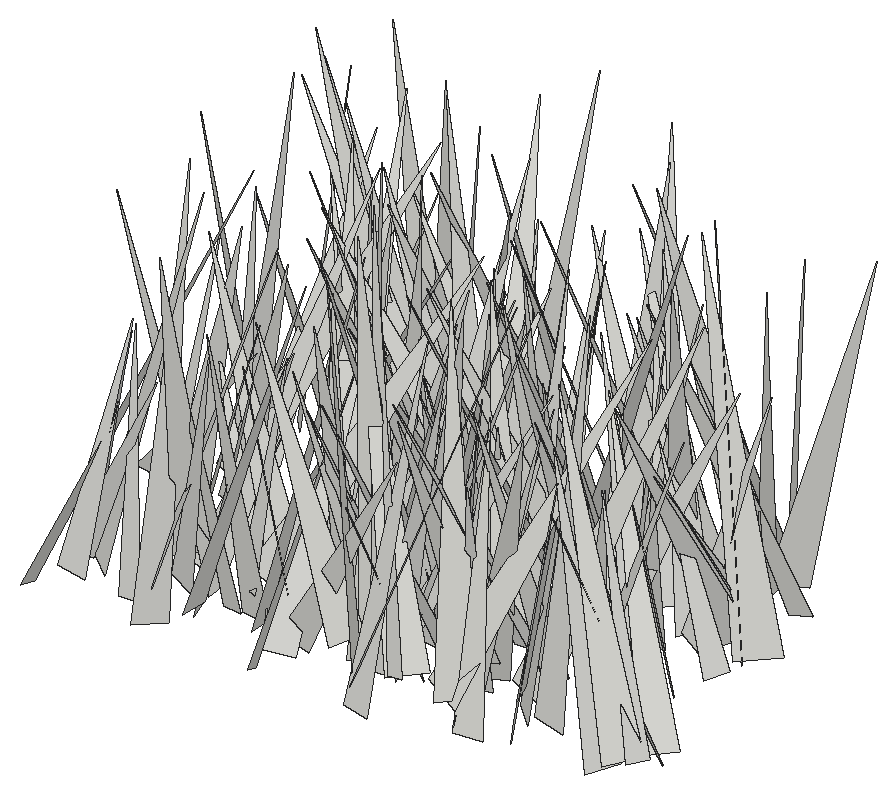
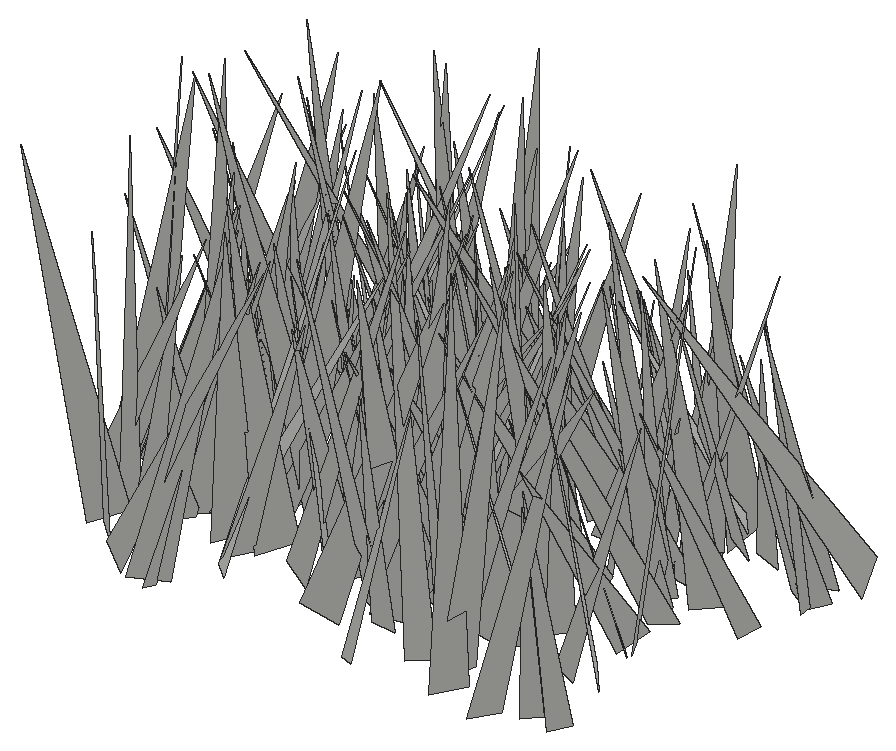
# SketchUp Ruby script. Lengths in inches.
U = 1.inch
M = Sketchup.active_model
def pt(a) = Geom::Point3d.new(a.map { |v| v * U })
def face(e, loops, mat)
  f = e.add_face(loops[0].map { |a| pt(a) })
  loops[1..].each { |l| e.add_face(l.map { |a| pt(a) }).erase! }
  f.material = f.back_material = mat if mat
  f
end
# faces: each face lists its corners as indices into pts; further lists are holes
def faces(e, pts, list, mat = nil) = list.each { |f| face(e, (f[0].is_a?(Array) ? f : [f]).map { |l| l.map { |i| pts[i] } }, mat) }
# xy, xz, yz: faces in a plane at the given z, y or x. An outline is a flat list of corners, or four numbers for a rectangle; further outlines are holes
def ring(l) = l.size == 4 ? [[l[0], l[1]], [l[2], l[1]], [l[2], l[3]], [l[0], l[3]]] : l.each_slice(2).to_a
def flat(e, list, mat, &to3) = list.each { |f| face(e, (f[0].is_a?(Array) ? f : [f]).map { |l| ring(l).map { |u, v| to3.(u, v) } }, mat) }
def xy(e, z, list, mat = nil) = flat(e, list, mat) { |x, y| [x, y, z] }
def xz(e, y, list, mat = nil) = flat(e, list, mat) { |x, z| [x, y, z] }
def yz(e, x, list, mat = nil) = flat(e, list, mat) { |y, z| [x, y, z] }
def lines(e, pts, list) = list.each { |a, b| e.add_line(pt(pts[a]), pt(pts[b])) }
# prism: a flat outline (further loops are holes) pulled along v
def prism(e, loops, v, mat = nil)
  f = face(e, loops, mat); d = Geom::Vector3d.new(v.map { |x| x * U })
  f.pushpull(f.normal.samedirection?(d) ? d.length : -d.length)
end
def box(e, o, s, mat = nil) = prism(e, [[o, [o[0] + s[0], o[1], o[2]], [o[0] + s[0], o[1] + s[1], o[2]], [o[0], o[1] + s[1], o[2]]]], [0, 0, s[2]], mat)
def at(x, y, z, deg = 0) = Geom::Transformation.translation(pt([x, y, z])) * Geom::Transformation.rotation(ORIGIN, Z_AXIS, deg.degrees)
def axes(o, x, y, z) = Geom::Transformation.new([*x, 0, *y, 0, *z, 0, *pt(o).to_a, 1])
def part(name) = M.definitions.add(name)
# library, detail: a bought-in or finely detailed component or shape, given as its bounding box
def library(name, o, s) = part(name).tap { |d| box(d.entities, o, s) }
def detail(e, o, s) = box(e.add_group.entities, o, s)
def put(e, d, t, mat = nil) = e.add_instance(d, t).tap { |i| i.material = mat if mat }
def group(e, t, mat = nil) = e.add_group.tap { |g| g.transformation = t; g.material = mat if mat }.entities
root = M.entities
c1 = part("fur_instance\#9")
p = [[0.8125,0,1.79],[0.67,-0.02,1.48],[0,-0.11,0],[0,0.11,0]]
faces(c1.entities,p,[[0,1,2,3]])
put(root,c1,axes([118.43,200.45,-27.1],[6.55283,1.12937,1.12544],[0.97488,-6.60494,0.95181],[-1.26162,0.76214,6.58096]))
put(root,c1,axes([128.43,203.72,-27.1],[1.50349,-5.86365,0.5049],[-5.82358,-1.55753,-0.74685],[-0.85041,0.2992,6.00709]))
put(root,c1,axes([121.35,202.26,-28.22],[2.07826,-5.21506,0.82935],[-4.82149,-1.51054,2.58366],[2.15357,1.65083,4.98405]))
put(root,c1,axes([123.91,201.99,-27.1],[-5.32926,2.77314,1.19327],[2.9808,5.21718,1.1879],[0.47858,-1.6143,5.88899]))
put(root,c1,axes([126.07,203.33,-28.22],[-2.66612,-3.28273,0.28859],[-3.19335,2.6653,0.81637],[0.81369,-0.29607,4.14946]))
put(root,c1,axes([126.01,199.82,-28.22],[2.11808,6.39246,0.96016],[6.39192,-2.22182,0.69185],[-0.96378,-0.68681,6.6986]))
put(root,c1,axes([131.1,202.04,-28.22],[4.62058,2.87983,1.50344],[3.15499,-4.60106,-0.88304],[-0.77446,-1.56215,5.37246]))
put(root,c1,axes([136.55,201.3,-27.1],[-5.76808,3.66085,1.08427],[3.77252,5.76709,0.59739],[0.58783,-1.08949,6.80556]))
put(root,c1,axes([129.43,201.09,-27.1],[-5.69,4.35692,2.08043],[4.49689,5.95288,-0.16772],[1.75752,-1.1258,7.16454]))
put(root,c1,axes([119.28,202.8125,-28.22],[-0.73911,-5.79285,1.55471],[-5.99778,0.70592,-0.22109],[-0.03032,1.57006,5.83563]))
put(root,c1,axes([125.12,201.11,-28.22],[-6.49961,-2.89491,2.26898],[-3.37847,6.5202,-1.35892],[1.4542,2.20912,6.98418]))
put(root,c1,axes([115.99,203.56,-27.1],[4.78165,-4.93816,1.39024],[-4.88475,-4.96331,-0.82896],[-1.56762,0.40313,6.82367]))
put(root,c1,axes([112.33,201.38,-28.22],[0.08637,4.97569,1.67082],[5.15736,0.22998,-0.95146],[0.97504,-1.65717,4.88463]))
put(root,c1,axes([130.11,200.84,-28.22],[-0.17119,5.69768,1.30234],[5.83131,0.07859,0.42267],[-0.39436,-1.31119,5.68456]))
put(root,c1,axes([135.11,201.98,-28.22],[-5.24229,2.67543,1.59997],[2.88849,5.34612,0.52444],[1.17239,-1.20849,5.86212]))
put(root,c1,axes([125.73,200.1,-27.1],[6.75975,3.62956,0.52461],[3.54067,-6.74583,1.04905],[-0.95528,0.68056,7.60048]))
put(root,c1,axes([136.04,203.83,-28.22],[-3.22391,-4.50813,0.36238],[-4.51102,3.23719,0.13952],[0.32445,0.21334,5.54053]))
put(root,c1,axes([115.06,201.15,-28.22],[0.59003,4.76484,1.13067],[4.77949,-0.80843,0.91275],[-1.06703,-0.9864,4.71367]))
put(root,c1,axes([117.36,202.06,-28.22],[4.51759,1.55237,1.02195],[1.60919,-4.61101,-0.10928],[-0.92991,-0.4377,4.77562]))
put(root,c1,axes([115.81,203.07,-28.22],[-0.90647,-5.11686,1.80724],[-5.12934,1.40604,1.40817],[1.7715,1.45288,5.00209]))
put(root,c1,axes([111.72,202.58,-28.22],[2.80159,-3.67069,0.58517],[-3.61323,-2.51742,1.50747],[0.87232,1.36159,4.36468]))
put(root,c1,axes([129.96,205.05,-27.1],[-4.86076,-4.47494,0.06756],[-4.36579,4.76306,1.38194],[0.98465,-0.972,6.46083]))
put(root,c1,axes([127.02,201.38,-27.1],[-4.60264,5.20733,0.96805],[5.29634,4.53648,0.77902],[0.04773,-1.24166,6.90606]))
put(root,c1,axes([111.87,202.94,-28.22],[5.07227,1.20948,1.05659],[1.39553,-5.05165,-0.91676],[-0.7948,-1.15114,5.13326]))
put(root,c1,axes([128.25,203.69,-28.22],[1.54796,-4.76639,0.70367],[-4.81569,-1.50748,0.38266],[0.1508,0.78667,4.99682]))
put(root,c1,axes([118.28,202.76,-28.22],[-1.858,-4.3991,1.45242],[-4.62148,1.65138,-0.9103],[-0.32175,1.68364,4.68782]))
put(root,c1,axes([127.35,203.25,-27.1],[-2.08811,-4.65792,0.59921],[-4.45757,1.75934,-1.85749],[-1.47829,1.27435,4.7546]))
put(root,c1,axes([124.63,203.15,-27.1],[-4.81324,5.46383,3.73935],[6.29264,5.21276,0.48307],[2.05886,-3.15867,7.26549]))
put(root,c1,axes([121.36,199.98,-28.22],[4.83042,2.64277,1.00625],[2.0268,-4.62442,2.4159],[-1.97202,1.72053,4.9478]))
put(root,c1,axes([124.89,203.09,-28.22],[5.25974,-3.61511,1.15521],[-3.73911,-5.27428,0.51907],[-0.65007,1.0869,6.36116]))
put(root,c1,axes([126.47,200.94,-27.1],[1.43872,7.93621,2.15807],[7.82752,-1.99366,2.11323],[-2.52399,-1.65906,7.7838]))
put(root,c1,axes([136.99,201.56,-27.1],[-4.67353,1.04438,0.03845],[1.02272,4.60667,-0.8165],[0.21505,0.78861,4.71868]))
put(root,c1,axes([133.02,201.65,-27.1],[2.04699,7.14679,2.15899],[7.40344,-2.23185,0.36858],[-0.96272,-1.9673,7.42502]))
put(root,c1,axes([128.07,204.48,-28.22],[4.17782,-5.39394,0.17375],[-5.37681,-4.14138,0.71959],[0.46328,0.57738,6.78461]))
put(root,c1,axes([123.94,202.81,-28.22],[-2.98009,3.50221,2.17702],[3.82104,3.35523,-0.16707],[1.55067,-1.53712,4.59549]))
put(root,c1,axes([116.65,200.26,-28.22],[-7.79963,1.89477,1.60693],[1.33324,7.65978,-2.56065],[2.09639,2.17814,7.60707]))
put(root,c1,axes([129.51,201.4375,-28.22],[5.12063,-0.00436,1.95562],[-0.62511,-5.19742,1.62522],[-1.85303,1.74129,4.85588]))
put(root,c1,axes([118.97,202.68,-27.1],[1.57919,4.13225,1.33364],[4.34025,-1.54395,-0.35548],[-0.12772,-1.37428,4.40942]))
put(root,c1,axes([127.67,203.25,-27.1],[4.70905,2.28139,1.77217],[2.5251,-4.89691,-0.40574],[-1.40329,-1.15586,5.21682]))
put(root,c1,axes([128.81,201.05,-27.1],[2.72489,7.5123,0.23605],[7.26372,-2.56761,-2.13568],[1.931,-0.94238,7.70056]))
put(root,c1,axes([112.57,202.55,-28.22],[4.61104,6.12434,1.67223],[6.3457,-4.50796,-0.9879],[-0.18966,-1.93296,7.60219]))
put(root,c1,axes([127.52,203.83,-28.22],[2.0151,-5.02328,1.60572],[-5.27188,-1.87389,0.75376],[0.13771,1.76848,5.35965]))
put(root,c1,axes([130.98,204.51,-27.1],[-0.18696,-5.47828,1.21386],[-5.53827,-0.01495,-0.92048],[-0.90141,1.22808,5.40363]))
put(root,c1,axes([123.99,203.75,-28.22],[-5.21279,-1.15752,0.50027],[-1.17064,5.23306,-0.0898],[0.46875,0.19648,5.33901]))
put(root,c1,axes([121.95,205.01,-28.22],[1.37866,-6.43403,1.32521],[-6.55871,-1.42426,-0.09169],[-0.36909,1.27608,6.57944]))
put(root,c1,axes([124.95,205.11,-28.22],[1.49707,-8.01218,1.60299],[-8.01526,-1.12338,1.87068],[1.58751,1.88383,7.93327]))
put(root,c1,axes([111.63,199.87,-28.22],[7.75154,3.11882,0.30174],[2.75499,-7.16733,3.30818],[-1.4927,2.96765,7.67264]))
put(root,c1,axes([116.23,200.82,-27.1],[4.52328,4.39752,0.22155],[4.10164,-4.32376,2.0806],[-1.60118,1.34692,5.95561]))
put(root,c1,axes([123.45,205.42,-27.1],[-3.4189,-2.83051,0.24342],[-2.77437,3.40847,0.66713],[0.61145,-0.36118,4.38812]))
put(root,c1,axes([117.02,203.63,-28.22],[-7.20158,-1.52489,0.67202],[-1.60184,7.15641,-0.92717],[0.45935,1.04894,7.30263]))
put(root,c1,axes([118.75,205.14,-28.22],[-3.29784,-3.61715,1.25797],[-3.53735,3.51322,0.8285],[1.46745,0.33986,4.82422]))
put(root,c1,axes([121.39,201.36,-28.22],[-3.94963,4.34285,0.40783],[4.0226,3.83915,-1.92507],[1.68683,1.01332,5.54563]))
put(root,c1,axes([125.86,205.01,-28.22],[-4.11377,-6.51171,1.45116],[-6.65439,3.88319,-1.43913],[-0.47668,1.98739,7.56666]))
put(root,c1,axes([125.12,204.41,-27.1],[2.82245,-3.27125,1.23973],[-3.47956,-2.78972,0.56063],[-0.36142,1.31172,4.28404]))
put(root,c1,axes([119.73,202.45,-28.22],[6.46332,2.41268,1.62775],[2.03661,-6.58136,1.66821],[-2.07914,1.05343,6.69422]))
put(root,c1,axes([130.66,203.27,-28.22],[4.76999,5.26227,1.90717],[5.37132,-5.00824,0.38463],[-1.57405,-1.14351,7.09199]))
put(root,c1,axes([128.39,202.98,-28.22],[2.68207,4.86571,0.6841],[4.89534,-2.71316,0.10499],[-0.42283,-0.54794,5.55496]))
put(root,c1,axes([121.53,204.46,-28.22],[-1.05184,5.80364,2.59591],[6.34975,1.09094,0.13387],[0.3189,-2.57972,5.89666]))
put(root,c1,axes([130.91,202.77,-27.1],[6.22186,3.72093,2.03459],[3.43335,-6.54009,1.46143],[-2.48938,0.27987,7.10078]))
put(root,c1,axes([127.45,205.02,-27.1],[-3.50463,1.38607,1.3282],[1.66931,3.56562,0.68373],[0.94799,-1.15452,3.70623]))
put(root,c1,axes([115.04,202.63,-27.1],[2.36342,5.34352,0.74133],[5.25737,-2.46286,0.99138],[-1.20944,-0.26392,5.75813]))
put(root,c1,axes([114.99,205.15,-27.1],[4.88196,1.64498,0.71636],[1.77456,-4.73338,-1.22423],[-0.26474,-1.39349,5.00407]))
put(root,c1,axes([128.9,205.42,-27.1],[-1.8038,-4.78632,0.84713],[-4.75617,1.55162,-1.36069],[-1.00264,1.25053,4.93062]))
put(root,c1,axes([131.8,207.57,-27.1],[-2.90473,-5.90083,0.221],[-5.68544,2.86131,1.67173],[1.5951,-0.54696,6.36102]))
put(root,c1,axes([125.35,202.85,-28.22],[5.3948,4.35682,0.5893],[4.31887,-5.42625,0.57994],[-0.82254,0.08385,6.9101]))
put(root,c1,axes([125.07,203.8125,-27.1],[2.90433,5.023,0.38727],[4.82562,-2.64532,-1.87916],[1.44702,-1.25991,5.48948]))
put(root,c1,axes([130.7,204.83,-28.22],[3.01328,1.01562,1.71575],[1.06477,-3.44849,0.1713],[-1.68569,-0.36275,3.17522]))
put(root,c1,axes([131.39,206.14,-27.1],[0.93641,-4.49496,0.58968],[-4.44892,-0.79539,1.00188],[0.87152,0.76939,4.48082]))
put(root,c1,axes([131.85,204.95,-28.22],[4.42305,4.26534,0.99754],[4.37397,-4.22348,-1.33498],[0.23791,-1.64944,5.99786]))
put(root,c1,axes([123.19,205.13,-27.1],[5.83146,1.27805,1.15338],[1.33487,-5.92923,-0.17895],[-1.08712,-0.42484,5.96719]))
put(root,c1,axes([118.87,204.97,-27.1],[-2.86629,5.19134,1.30889],[5.27356,2.48156,1.70596],[-0.92348,-1.94182,5.67938]))
put(root,c1,axes([128.82,208.22,-27.1],[-3.40543,-6.99905,0.02732],[-6.9991,3.40539,-0.01642],[-0.00281,0.03175,7.78353]))
put(root,c1,axes([126.48,206.82,-27.1],[-3.7934,-3.57067,0.95546],[-3.47781,3.9116,0.81037],[1.25196,0.04698,5.14615]))
put(root,c1,axes([119.21,203.48,-27.1],[-0.59602,7.49567,1.64856],[6.68012,1.32078,-3.59019],[3.77872,-1.15261,6.60687]))
put(root,c1,axes([135.98,204.0625,-28.22],[-2.5947,5.83184,0.30944],[5.66182,2.42897,1.69778],[-1.43174,-0.96349,6.15308]))
put(root,c1,axes([117.38,205.2,-28.22],[-2.80157,3.07223,0.58027],[3.12461,2.72376,0.66487],[-0.11008,-0.87559,4.10431]))
put(root,c1,axes([134.82,206.15,-27.1],[-2.53419,-2.69204,0.92744],[-2.77792,2.61003,-0.01451],[0.6248,0.68554,3.69715]))
put(root,c1,axes([115.08,206.99,-27.1],[1.45023,-6.39796,1.08768],[-6.25164,-1.07813,1.99368],[1.74182,1.45734,6.24998]))
put(root,c1,axes([129.87,208.44,-27.1],[2.52782,-6.77606,0.30453],[-6.73549,-2.54598,-0.74076],[-0.80053,0.02468,7.19418]))
put(root,c1,axes([129.96,204.41,-28.22],[1.6055,7.88479,1.47704],[7.72527,-1.11383,-2.45126],[2.16141,-1.87581,7.66412]))
put(root,c1,axes([113.36,206.51,-27.1],[2.93008,-5.46925,1.49234],[-5.65269,-2.69042,1.23848],[0.43226,1.89052,6.07982]))
put(root,c1,axes([116.31,205.49,-27.1],[1.54209,5.92638,1.72605],[6.04197,-1.81335,0.82809],[-1.2633,-1.43843,6.06748]))
put(root,c1,axes([132.16,205.22,-27.1],[-1.31854,4.49628,0.43937],[4.51767,1.31381,0.11263],[0.01505,-0.45333,4.68427]))
put(root,c1,axes([114.54,207.59,-27.1],[1.31964,-4.20384,0.49444],[-3.9297,-1.02429,1.77946],[1.57296,0.96785,4.03079]))
put(root,c1,axes([111.18,206.97,-27.1],[2.58418,-3.37784,0.00054],[-2.92311,-2.23595,2.1316],[1.69269,1.29557,3.68023]))
put(root,c1,axes([127.53,206.46,-27.1],[-3.57367,4.96866,1.72232],[5.21894,3.60663,0.42422],[0.64547,-1.65218,6.10563]))
put(root,c1,axes([116.01,204.21,-28.22],[2.50136,7.65725,0.1478],[7.63522,-2.48107,-0.67805],[0.59891,-0.35058,8.02686]))
put(root,c1,axes([133.32,206.43,-27.1],[-5.60882,2.54428,1.1021],[2.59069,5.69507,0.03704],[0.9881,-0.48955,6.15881]))
put(root,c1,axes([132.29,208.24,-27.1],[0.84886,-4.32385,0.54485],[-4.30912,-0.7498,0.76315],[0.65118,0.6747,4.3398]))
put(root,c1,axes([132.6,206.29,-27.1],[-3.91577,-3.49387,3.17429],[-4.26524,4.38586,-0.43413],[2.02262,2.48468,5.2299]))
put(root,c1,axes([122.07,206.52,-27.1],[-0.00345,4.9845,1.60202],[5.18158,-0.22632,0.71534],[-0.75028,-1.58596,4.93291]))
put(root,c1,axes([134.37,210.35,-27.1],[4.00993,-5.51552,0.33203],[-5.14979,-3.87921,-2.24547],[-2.00271,-1.06842,6.43882]))
put(root,c1,axes([128.66,209.22,-27.1],[-6.87561,-0.89332,0.66489],[-0.69538,6.69239,1.80069],[0.86979,-1.71115,6.69549]))
put(root,c1,axes([131.08,206.76,-27.1],[0.63179,6.0642,2.01169],[5.81387,0.29266,-2.70812],[2.6496,-2.08816,5.46258]))
put(root,c1,axes([126.26,208.2,-27.1],[-2.43401,-4.94438,0.27236],[-4.40728,2.02468,-2.63096],[-2.25763,1.37813,4.84245]))
put(root,c1,axes([125.18,208.46,-27.1],[2.03296,-3.43324,0.36978],[-3.45285,-2.01606,0.26469],[0.04074,0.45292,3.9812]))
put(root,c1,axes([130.52,209.08,-27.1],[-1.29347,-4.18784,0.40951],[-4.17089,1.33267,0.45438],[0.55623,0.25449,4.35943]))
put(root,c1,axes([123.68,207.34,-27.1],[5.7925,1.49056,1.34896],[1.52882,-5.93778,-0.00376],[-1.30544,-0.3399,5.9812]))
put(root,c1,axes([120.92,207.74,-27.1],[-2.66914,2.15187,1.53787],[2.38339,2.90414,0.07299],[1.14676,-1.02728,3.42776]))
put(root,c1,axes([131.25,207.51,-27.1],[-2.34168,-2.41248,1.9117],[-2.76899,2.70012,0.01564],[1.3444,1.35921,3.36204]))
put(root,c1,axes([135.36,207.93,-27.1],[-3.9914,1.89648,0.82188],[2.01712,3.964,0.64912],[0.45094,-0.94526,4.3711]))
put(root,c1,axes([122.61,209.625,-27.1],[-0.7364,-6.55979,0.93298],[-6.36781,0.44127,-1.92351],[-1.83094,1.10364,6.31453]))
put(root,c1,axes([123.43,207.78,-27.1],[-1.82115,-3.36265,1.61921],[-3.73204,1.65736,-0.7556],[0.03439,1.7865,3.74875]))
put(root,c1,axes([120.5,207.69,-27.1],[4.06784,5.47307,2.7985],[5.78633,-4.54195,0.47187],[-2.07475,-1.93641,6.80288]))
put(root,c1,axes([127.06,206.29,-27.1],[-6.05954,0.33778,0.89505],[0.02694,5.79744,-2.00555],[0.95629,1.97708,5.728]))
put(root,c1,axes([125.32,208.01,-27.1],[-1.86227,-3.58892,1.59018],[-3.91628,1.57852,-1.02377],[-0.26793,1.87217,3.91156]))
put(root,c1,axes([134.66,211.29,-27.1],[-4.06772,-3.26977,0.32403],[-2.78571,3.7053,2.41936],[1.74246,-1.70943,4.62433]))
put(root,c1,axes([119.39,207.26,-27.1],[1.43263,3.39143,0.32506],[3.34277,-1.46736,0.57677],[-0.65831,-0.07043,3.63615]))
put(root,c1,axes([123.82,209.55,-27.1],[4.04014,-3.74392,1.13553],[-3.80741,-4.13804,-0.09691],[-0.90002,0.69913,5.50729]))
put(root,c1,axes([113.61,210.21,-27.1],[-6.01698,-4.0059,2.23214],[-3.85326,6.41302,1.12219],[2.48637,0.24439,7.14087]))
put(root,c1,axes([127.23,207.82,-27.1],[1.06492,5.99669,1.55027],[6.17359,-1.15473,0.22589],[-0.50038,-1.48458,6.08632]))
put(root,c1,axes([122.11,209.9,-27.1],[-5.99234,-4.15881,0.58341],[-4.19764,5.96205,-0.6148],[0.12593,0.83815,7.26814]))
put(root,c1,axes([119.22,207.13,-27.1],[-5.83364,4.02968,1.05878],[3.90844,5.92385,-1.01134],[1.44341,0.24573,7.01761]))
put(root,c1,axes([120.09,207.83,-27.1],[-5.57386,3.34507,0.61319],[3.34749,5.6042,-0.14346],[0.5998,-0.19191,6.49898]))
put(root,c1,axes([118.17,209.3,-27.1],[5.45486,-2.53583,1.72286],[-2.73109,-5.61705,0.37948],[-1.39279,1.08278,6.00349]))
put(root,c1,axes([126.59,210.05,-27.1],[0.40641,-5.35004,1.66525],[-5.54368,-0.62666,-0.66032],[-0.81458,1.59547,5.32467]))
put(root,c1,axes([115.12,207.05,-27.1],[-7.30658,0.78889,2.52937],[0.00726,7.42557,-2.29501],[2.64953,2.15518,6.98151]))
put(root,c1,axes([126.48,210.55,-27.1],[4.42301,-0.66017,1.25029],[-0.31732,-4.46498,-1.23502],[-1.37781,-1.09094,4.29808]))
put(root,c1,axes([123.5,210.72,-27.1],[-6.69596,1.51903,0.23584],[1.52209,6.40398,1.96756],[-0.2152,-1.96993,6.57815]))
put(root,c1,axes([123.33,206.8,-27.1],[1.15921,7.66569,0.40932],[7.66684,-1.17697,0.3294],[-0.3873,-0.35503,7.74584]))
put(root,c1,axes([125.68,209.01,-27.1],[2.94995,3.39967,1.09614],[3.50655,-3.02709,-0.04841],[-0.68072,-0.86052,4.50085]))
put(root,c1,axes([116.93,207.73,-27.1],[5.85572,0.96623,0.0245],[0.91904,-5.61274,1.69591],[-0.29926,1.66948,5.68743]))
put(root,c1,axes([120.04,209.72,-27.1],[-0.77614,4.62516,2.62163],[4.88719,1.66369,-1.48826],[2.09294,-2.16967,4.44742]))
put(root,c1,axes([130.79,211.92,-27.1],[0.39282,-7.92697,1.06347],[-7.86049,-0.18606,1.51663],[1.47665,1.11832,7.79044]))
put(root,c1,axes([127.57,209.76,-27.1],[8.28106,0.30024,0.90595],[0.31898,-8.32832,-0.15571],[-0.89952,-0.18935,8.28504]))
put(root,c1,axes([133.2,209.17,-27.1],[2.00403,4.77087,1.2081],[4.88814,-1.77806,-1.08691],[0.57161,-1.52123,5.05925]))
put(root,c1,axes([116.21,211.08,-27.1],[5.02867,-2.50397,0.95955],[-2.41233,-5.11484,-0.70513],[-1.17101,-0.21602,5.57317]))
put(root,c1,axes([128.75,210.77,-27.1],[-2.94744,-5.34651,0.76174],[-5.29498,2.69026,-1.60576],[-1.06233,1.42484,5.89017]))
put(root,c1,axes([135.75,209.7,-27.1],[-4.55755,6.1935,2.40469],[6.62517,4.45559,1.08074],[0.49905,-2.58872,7.61332]))
put(root,c1,axes([135.03,209.61,-27.1],[-5.85102,-5.01294,3.05498],[-5.59861,6.06235,-0.77491],[1.76582,2.61061,7.66574]))
put(root,c1,axes([113.83,208.32,-27.1],[1.59933,7.72158,1.03232],[7.26868,-1.09996,-3.03359],[2.80263,-1.55359,7.2786]))
put(root,c1,axes([120.22,210.22,-27.1],[4.77754,4.17311,2.72058],[4.61145,-5.13068,-0.22808],[-1.8844,-1.97551,6.33938]))
put(root,c1,axes([119.35,207.38,-27.1],[-1.39232,7.88876,0.40308],[7.89477,1.37627,0.33483],[-0.26016,-0.45487,8.00369]))
put(root,c1,axes([118.83,211.41,-27.1],[0.4901,-6.09421,1.40714],[-6.12992,-0.18765,1.32232],[1.24239,1.47818,5.96918]))
put(root,c1,axes([120.79,208.34,-27.1],[-3.36626,3.2291,1.55087],[2.48228,3.63709,-2.18492],[2.58275,0.71309,4.12128]))
put(root,c1,axes([131.17,207.81,-27.1],[3.09687,5.17866,0.3937],[4.90573,-3.06729,1.75775],[-1.70508,0.58082,5.7723]))
put(root,c1,axes([132.82,209.9,-27.1],[-6.31107,2.62453,1.38258],[2.63294,6.45317,-0.23139],[1.36651,-0.31261,6.83112]))
put(root,c1,axes([122.08,211.03,-27.1],[2.26565,-5.57265,3.25786],[-5.77256,-3.29433,-1.62055],[-2.88887,2.21229,5.79322]))
put(root,c1,axes([113.57,210.74,-27.1],[3.56732,3.05528,0.6125],[3.0981,-3.37772,-1.19517],[0.33415,-1.30074,4.54225]))
put(root,c1,axes([123.37,210.1,-27.1],[-7.4138,3.10521,1.79195],[3.13289,7.61249,-0.22981],[1.74312,-0.47482,8.03455]))
put(root,c1,axes([122.11,209.05,-27.1],[-0.74484,5.04348,0.31723],[4.84937,0.80355,-1.38926],[1.42161,-0.09859,4.90524]))
put(root,c1,axes([121.17,212.28,-27.1],[2.55159,-4.81811,0.15811],[-4.66384,-2.42197,1.46026],[1.21971,0.81832,5.25284]))
put(root,c1,axes([116.51,212.39,-27.1],[4.04472,-2.80495,1.23292],[-2.68281,-4.22845,-0.81868],[-1.47998,-0.00072,4.85358]))
put(root,c1,axes([130.94,210.61,-27.1],[-3.74669,3.50171,1.17991],[3.59906,3.83892,0.03541],[0.8372,-0.8322,5.12819]))
put(root,c1,axes([129.78,211.55,-27.1],[-5.18196,-4.15409,0.26027],[-4.02731,4.89921,-1.98883],[-1.05116,1.70828,6.3367]))
put(root,c1,axes([125.33,211.26,-27.1],[-5.00491,-0.78513,1.46412],[-0.94309,5.16869,-0.45214],[1.36772,0.69095,5.0459]))
put(root,c1,axes([117.93,210.06,-27.1],[-5.27031,-0.93158,1.82448],[-1.52104,5.15288,-1.7627],[1.37223,2.13373,5.05341]))
put(root,c1,axes([121.33,213.91,-27.1],[3.93068,-5.30389,1.53813],[-4.85639,-4.21869,-2.1367],[-2.62918,-0.13704,6.24628]))
put(root,c1,axes([132.51,213.28,-27.1],[3.93846,-2.19121,0.70559],[-1.95473,-3.92185,-1.26841],[-1.21585,-0.79274,4.32481]))
put(root,c1,axes([134.93,213.03,-27.1],[-0.6126,-5.21006,0.97224],[-5.10965,0.32064,-1.50131],[-1.40764,1.1035,5.02654]))
put(root,c1,axes([127.97,214.875,-27.1],[-5.57338,-5.53642,0.81265],[-5.27737,5.58191,1.83481],[1.86058,-0.75178,7.63858]))
put(root,c1,axes([124.06,212.35,-27.1],[-6.12139,2.10353,0.29479],[2.12072,6.0019,1.20952],[-0.1196,-1.23917,6.35872]))
put(root,c1,axes([131.29,212.88,-27.1],[-5.2528,1.04607,1.18822],[1.28573,5.22141,1.0871],[0.92359,-1.31932,5.24446]))
put(root,c1,axes([131.82,212.81,-27.1],[-5.37487,-0.5228,0.79074],[-0.44432,5.41107,0.55741],[0.83736,-0.48456,5.37139]))
put(root,c1,axes([114.31,213.18,-27.1],[-1.82389,-4.57282,0.8897],[-4.65371,1.74485,-0.5721],[-0.21262,1.03617,4.88978]))
put(root,c1,axes([133.42,213.09,-27.1],[6.36794,0.62079,2.33056],[0.97414,-6.68136,-0.88201],[-2.20634,-1.15823,6.33704]))
put(root,c1,axes([123.21,211.3125,-27.1],[-4.28711,2.60894,1.39768],[2.40918,4.50508,-1.01958],[1.71929,0.19268,4.91389]))
put(root,c1,axes([119.54,211.93,-27.1],[3.95352,-1.35205,0.74696],[-1.51739,-3.78343,1.18299],[-0.28899,1.3689,4.00736]))
put(root,c1,axes([118.78,215.49,-27.1],[8.12463,-0.31909,0.21051],[-0.21684,-7.53553,-3.0536],[-0.31483,-3.04462,7.53571]))
put(root,c1,axes([123.47,215.13,-27.1],[0.28426,-7.43419,0.75555],[-7.30944,-0.43371,-1.51752],[-1.55247,0.68085,7.28321]))
put(root,c1,axes([125.8,213.49,-27.1],[-3.53449,-6.31522,1.62159],[-6.50822,3.306,-1.31053],[-0.39309,2.04757,7.11738]))
put(root,c1,axes([125.5,211.4375,-27.1],[-4.48164,3.41054,1.04148],[3.17852,4.57879,-1.31654],[1.61662,0.45221,5.47573]))
put(root,c1,axes([131.28,212.37,-27.1],[-5.13567,3.95215,0.39173],[3.97037,5.09374,0.66187],[-0.09557,-0.76314,6.44644]))
put(root,c1,axes([123.96,213.81,-27.1],[4.93042,2.67254,1.54888],[2.99605,-4.84755,-1.1728],[-0.75178,-1.79146,5.48417]))
put(root,c1,axes([118.12,212.9,-27.1],[-2.53782,7.33959,2.16761],[7.45924,1.86167,2.42953],[-1.71111,-2.77006,7.37615]))
put(root,c1,axes([113.84,209.98,-27.1],[-4.95607,3.58078,0.35964],[3.00453,4.45388,-2.94106],[1.98095,2.2034,5.36049]))
put(root,c1,axes([120.14,212.39,-27.1],[-2.8355,7.09509,0.7949],[6.33308,2.10473,3.80453],[-3.2961,-2.05963,6.62616]))
put(root,c1,axes([127.45,212.47,-27.1],[5.828,-3.21448,3.45143],[-4.0564,-6.21538,1.06086],[-2.40642,2.69201,6.57061]))
put(root,c1,axes([122.92,211.39,-27.1],[-3.64093,6.72533,0.73654],[6.73348,3.68347,-0.34805],[0.65778,-0.48058,7.63972]))
put(root,c1,axes([118.45,214.04,-27.1],[-6.63907,0.80935,0.83748],[0.8673,6.67065,0.42894],[0.7773,-0.53025,6.67446]))
put(root,c1,axes([119.55,213.31,-27.1],[-5.60874,-1.91132,2.91151],[-2.48414,6.06379,-0.80475],[2.44113,1.77916,5.87056]))
put(root,c1,axes([128.22,213.67,-27.1],[-5.4054,2.23783,0.44972],[2.26041,5.40869,0.2551],[0.31726,-0.40826,5.84475]))
put(root,c1,axes([113.28,212.64,-27.1],[4.45887,4.52554,1.75159],[4.30275,-4.78695,1.41478],[-2.24387,-0.18639,6.19358]))
put(root,c1,axes([113.875,214.64,-27.1],[4.52674,3.32324,0.78926],[3.39525,-4.2348,-1.64226],[0.37301,-1.78348,5.37013]))
put(root,c1,axes([133.36,214.31,-27.1],[5.70203,-3.94241,1.833],[-4.2894,-5.59456,1.31056],[-0.70959,2.13867,6.80721]))
put(root,c1,axes([129.09,212.73,-27.1],[5.10712,-2.96498,5.20518],[-4.57955,-6.3419,0.88079],[-3.86171,3.59957,5.83935]))
put(root,c1,axes([129.23,217.25,-27.1],[-5.21619,-2.22313,1.39253],[-1.54183,5.10575,2.37575],[2.12232,-1.75473,5.14847]))
put(root,c1,axes([121.18,214.49,-27.1],[0.37459,4.6587,1.44665],[4.87681,-0.39143,-0.00226],[-0.11359,-1.44218,4.67373]))
put(root,c1,axes([120.75,217.07,-27.1],[-2.24525,-3.81491,0.32062],[-3.67914,2.25292,1.04201],[1.05843,-0.26136,4.3022]))
put(root,c1,axes([116.68,216.54,-27.1],[7.00851,-2.19777,2.01204],[-2.01969,-7.2848,-0.92211],[-2.19075,-0.31499,7.28692]))
put(root,c1,axes([129.54,216.91,-27.1],[4.80769,-4.80499,2.60276],[-4.52111,-5.44469,-1.70033],[-3.0695,0.49361,6.58109]))
put(root,c1,axes([132.78,215.125,-27.1],[3.82157,4.19761,2.25189],[4.45533,-4.17126,0.21447],[-1.68552,-1.50865,5.67259]))
put(root,c1,axes([117.2,215.49,-27.1],[-7.37907,1.498,2.27835],[1.63074,7.6926,0.22378],[2.18531,-0.6822,7.52626]))
put(root,c1,axes([121.88,213.86,-27.1],[2.95959,7.19025,1.54721],[7.29869,-3.07695,0.338],[-0.90704,-1.29822,7.76818]))
put(root,c1,axes([113.28,216.24,-27.1],[2.68413,-2.59886,0.79499],[-2.66781,-2.73276,0.07385],[-0.51851,0.60713,3.7354]))
put(root,c1,axes([112.07,216.22,-27.1],[3.6262,-2.26105,0.60128],[-2.31235,-3.63241,0.28605],[-0.35624,0.56255,4.26378]))
put(root,c1,axes([131.46,216.41,-27.1],[-4.03956,-5.75099,0.92293],[-5.66396,3.6166,-2.25467],[-1.3584,2.0224,6.65646]))
put(root,c1,axes([114.64,217.14,-27.1],[-6.49711,1.14641,2.18071],[1.63194,6.61021,1.38712],[1.84567,-1.80917,6.45001]))
